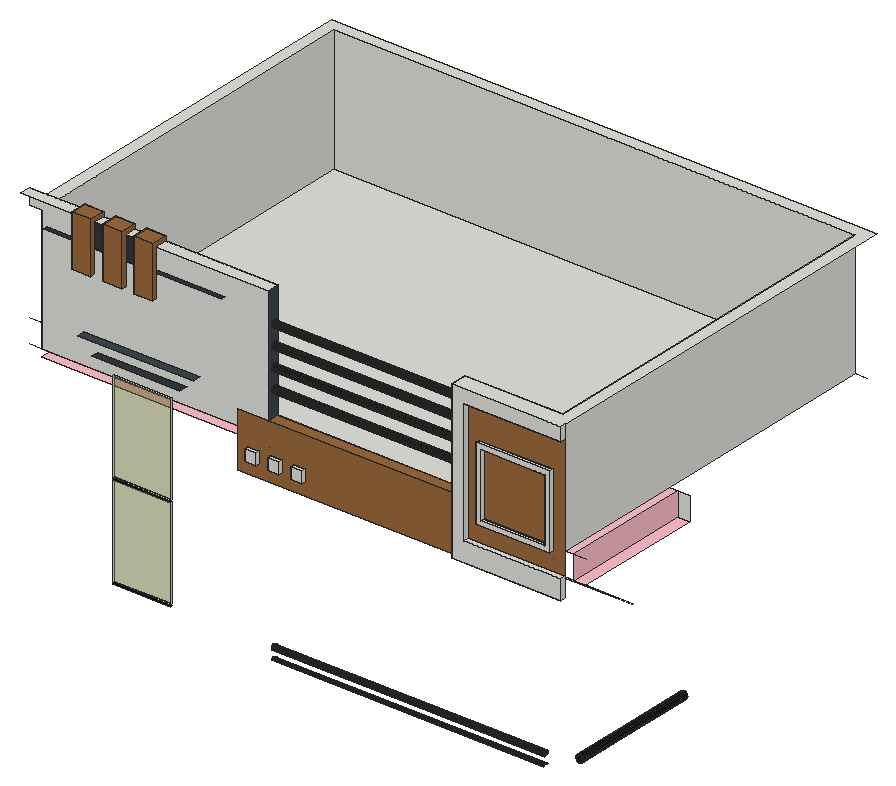
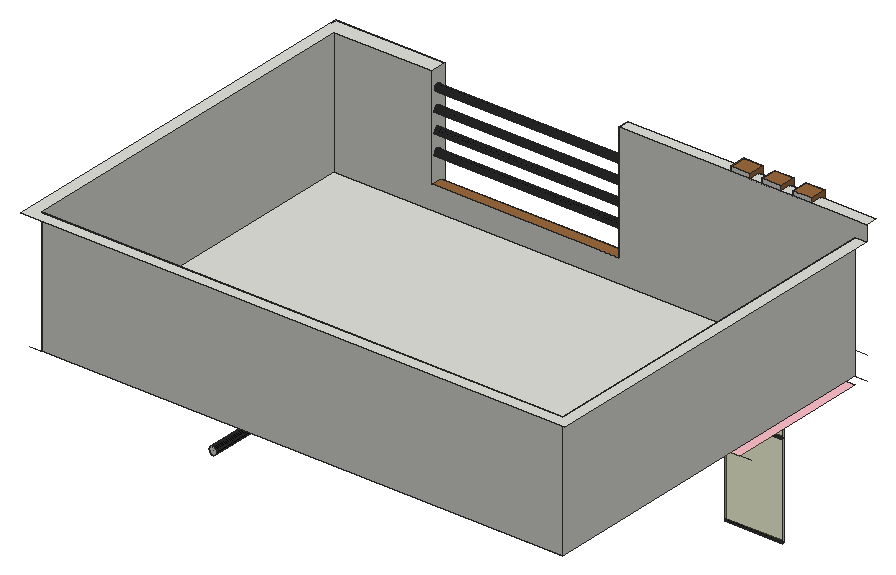
# SketchUp Ruby script. Lengths in inches.
U = 1.inch
M = Sketchup.active_model
def pt(a) = Geom::Point3d.new(a.map { |v| v * U })
def face(e, loops, mat)
  f = e.add_face(loops[0].map { |a| pt(a) })
  loops[1..].each { |l| e.add_face(l.map { |a| pt(a) }).erase! }
  f.material = f.back_material = mat if mat
  f
end
# faces: each face lists its corners as indices into pts; further lists are holes
def faces(e, pts, list, mat = nil) = list.each { |f| face(e, (f[0].is_a?(Array) ? f : [f]).map { |l| l.map { |i| pts[i] } }, mat) }
# xy, xz, yz: faces in a plane at the given z, y or x. An outline is a flat list of corners, or four numbers for a rectangle; further outlines are holes
def ring(l) = l.size == 4 ? [[l[0], l[1]], [l[2], l[1]], [l[2], l[3]], [l[0], l[3]]] : l.each_slice(2).to_a
def flat(e, list, mat, &to3) = list.each { |f| face(e, (f[0].is_a?(Array) ? f : [f]).map { |l| ring(l).map { |u, v| to3.(u, v) } }, mat) }
def xy(e, z, list, mat = nil) = flat(e, list, mat) { |x, y| [x, y, z] }
def xz(e, y, list, mat = nil) = flat(e, list, mat) { |x, z| [x, y, z] }
def yz(e, x, list, mat = nil) = flat(e, list, mat) { |y, z| [x, y, z] }
def lines(e, pts, list) = list.each { |a, b| e.add_line(pt(pts[a]), pt(pts[b])) }
# prism: a flat outline (further loops are holes) pulled along v
def prism(e, loops, v, mat = nil)
  f = face(e, loops, mat); d = Geom::Vector3d.new(v.map { |x| x * U })
  f.pushpull(f.normal.samedirection?(d) ? d.length : -d.length)
end
def box(e, o, s, mat = nil) = prism(e, [[o, [o[0] + s[0], o[1], o[2]], [o[0] + s[0], o[1] + s[1], o[2]], [o[0], o[1] + s[1], o[2]]]], [0, 0, s[2]], mat)
def at(x, y, z, deg = 0) = Geom::Transformation.translation(pt([x, y, z])) * Geom::Transformation.rotation(ORIGIN, Z_AXIS, deg.degrees)
def axes(o, x, y, z) = Geom::Transformation.new([*x, 0, *y, 0, *z, 0, *pt(o).to_a, 1])
def part(name) = M.definitions.add(name)
# library, detail: a bought-in or finely detailed component or shape, given as its bounding box
def library(name, o, s) = part(name).tap { |d| box(d.entities, o, s) }
def detail(e, o, s) = box(e.add_group.entities, o, s)
def put(e, d, t, mat = nil) = e.add_instance(d, t).tap { |i| i.material = mat if mat }
def group(e, t, mat = nil) = e.add_group.tap { |g| g.transformation = t; g.material = mat if mat }.entities
root = M.entities
M.materials.add("[0006_Pink]").color = [255, 192, 203]
M.materials.add("[0111_SlateGray]").color = [49, 56, 63]
M.materials.add("[0111_SlateGray]1").color = [61, 70, 79]
M.materials.add("[0137_Black]").color = [0, 0, 0]
M.materials.add("[Translucent Glass Gray]").color = [124, 128, 62]
M.materials["[Translucent Glass Gray]"].alpha = 0.5
M.materials.add("[Wood Floor]").color = [155, 105, 61]
xy(root,597.83,[[138.3,14,227.59,16]])
xy(root,600.83,[[138.3,14,227.59,16]])
xy(root,682.9,[[411.23,248,466.96,249],[473.67,248,530.59,249],[643.26,248,751.37,249]])
xy(root,741.83,[[138.3,14,227.59,16]])
xy(root,744.83,[[138.3,14,227.59,16]])
xy(root,828,[[821.4375,48.0625,840,248]],"[0006_Pink]")
xy(root,828,[[671.22,0,671.22,8,383.22,8,383.22,26,802.875,26,802.875,8,840,8,840,0]],"[Wood Floor]")
xy(root,847.68,[[350.63,2,368.01,8],[386.32,2,403.69,8],[421.88,2,439.26,8]])
xy(root,858,[[690.42,0,840,8]])
xy(root,864,[[407.75,124.89,404.625,125,401.625,125.91,398.97,127.5625,396.83,129.85,395.35,132.62,394.64,135.67,394.75,138.8,395.66,141.8,397.3125,144.45,399.6,146.59,402.37,148.07,405.42,148.78,408.55,148.67,411.55,147.76,414.2,146.11,416.34,143.82,417.82,141.06,418.53,138,418.42,134.875,417.51,131.875,415.86,129.22,413.57,127.08,410.81,125.6],[527.75,124.89,524.625,125,521.625,125.91,518.97,127.5625,516.83,129.85,515.35,132.62,514.64,135.67,514.75,138.8,515.66,141.8,517.3125,144.45,519.6,146.59,522.37,148.07,525.42,148.78,528.55,148.67,531.55,147.76,534.2,146.11,536.34,143.82,537.82,141.06,538.53,138,538.42,134.875,537.51,131.875,535.86,129.22,533.57,127.08,530.81,125.6],[647.75,124.89,644.625,125,641.625,125.91,638.97,127.5625,636.83,129.85,635.35,132.62,634.64,135.67,634.75,138.8,635.66,141.8,637.3125,144.45,639.6,146.59,642.37,148.07,645.42,148.78,648.55,148.67,651.55,147.76,654.2,146.11,656.34,143.82,657.82,141.06,658.53,138,658.42,134.875,657.51,131.875,655.86,129.22,653.57,127.08,650.81,125.6]])
xy(root,864,[[[18,26,18,248,821.4375,248,821.4375,48.0625,802.875,48.0625,802.875,26],[527.75,124.89,530.81,125.6,533.57,127.08,535.86,129.22,537.51,131.875,538.42,134.875,538.53,138,537.82,141.06,536.34,143.82,534.2,146.11,531.55,147.76,528.55,148.67,525.42,148.78,522.37,148.07,519.6,146.59,517.3125,144.45,515.66,141.8,514.75,138.8,514.64,135.67,515.35,132.62,516.83,129.85,518.97,127.5625,521.625,125.91,524.625,125],[647.75,124.89,650.81,125.6,653.57,127.08,655.86,129.22,657.51,131.875,658.42,134.875,658.53,138,657.82,141.06,656.34,143.82,654.2,146.11,651.55,147.76,648.55,148.67,645.42,148.78,642.37,148.07,639.6,146.59,637.3125,144.45,635.66,141.8,634.75,138.8,634.64,135.67,635.35,132.62,636.83,129.85,638.97,127.5625,641.625,125.91,644.625,125],[407.75,124.89,410.81,125.6,413.57,127.08,415.86,129.22,417.51,131.875,418.42,134.875,418.53,138,417.82,141.06,416.34,143.82,414.2,146.11,411.55,147.76,408.55,148.67,405.42,148.78,402.37,148.07,399.6,146.59,397.3125,144.45,395.66,141.8,394.75,138.8,394.64,135.67,395.35,132.62,396.83,129.85,398.97,127.5625,401.625,125.91,404.625,125]]],"[0006_Pink]")
xy(root,865.06,[[350.63,2,368.01,8],[386.32,2,403.69,8],[421.88,2,439.26,8]])
xy(root,876,[[18,26,822,590]])
xy(root,885.73,[[707.57,2,820.78,8]])
xy(root,885.83,[[138.3,14,227.59,16]])
xy(root,892.8,[[714.64,2,813.7,8]])
xy(root,909.62,[[114.5,2,251.38,14]],"[0111_SlateGray]")
xy(root,912,[[383.22,8,671.22,26]],"[Wood Floor]")
xy(root,930.88,[[93.24,2,272.64,14]],"[0111_SlateGray]1")
xy(root,991.86,[[714.64,2,813.7,8]])
xy(root,998.9375,[[707.57,2,820.78,8]])
xy(root,1020,[[85.01,1,114.04,8],[132.95,1,161.97,8],[180.58,1,209.6,8]])
xy(root,1047.6,[[690.42,0,840,8]])
xy(root,1056,[[36,8,311.22,14]],"[0111_SlateGray]")
xy(root,1068,[[671.22,0,840,0,840,608,0,608,0,26,18,26,18,590,822,590,822,26,671.22,26]])
xy(root,1092,[[0,8,85.01,26],[85.01,8,114.04,26],[114.04,8,132.95,26],[132.95,8,161.97,26],[161.97,8,180.58,26],
  [180.58,8,209.6,26],[209.6,8,383.22,26]])
xy(root,1099,[[85.01,1,114.04,26],[132.95,1,161.97,26],[180.58,1,209.6,26]],"[Wood Floor]")
xz(root,0,[[671.22,828,840,828,840,858,690.42,858,690.42,1047.6,840,1047.6,840,1068,671.22,1068]])
xz(root,1,[[85.01,1020,114.04,1099],[132.95,1020,161.97,1099],[180.58,1020,209.6,1099]],"[Wood Floor]")
xz(root,2,[[350.63,847.68,368.01,865.06],[386.32,847.68,403.69,865.06],[421.88,847.68,439.26,865.06],[[707.57,885.73,820.78,998.9375],[714.64,892.8,813.7,991.86]]])
xz(root,8,[[386.32,847.68,403.69,865.06],[421.88,847.68,439.26,865.06],[[707.57,885.73,820.78,998.9375],[714.64,892.8,813.7,991.86]],[85.01,1020,114.04,1056],[132.95,1020,161.97,1056],
  [180.58,1020,209.6,1056],[85.01,1056,114.04,1092],[132.95,1056,161.97,1092],[180.58,1056,209.6,1092]])
xz(root,8,[[114.04,1056,132.95,1092],[161.97,1056,180.58,1092]],"[0111_SlateGray]")
xz(root,8,[[[335.22,828,671.22,912],[350.63,847.68,368.01,865.06],[386.32,847.68,403.69,865.06],[421.88,847.68,439.26,865.06]],[[690.42,858,840,1047.6],[707.57,885.73,820.78,998.9375]],[714.64,892.8,813.7,991.86]],"[Wood Floor]")
xz(root,14,[[138.3,597.83,227.59,600.83],[138.3,741.83,227.59,744.83]],"[0137_Black]")
xz(root,16,[[138.3,600.83,227.59,741.83],[138.3,744.83,227.59,885.83]],"[Translucent Glass Gray]")
xz(root,26,[[383.22,828,802.875,864],[18,876,18,1068,0,1068,0,1092,383.22,1092,383.22,912,671.22,912,671.22,1068,822,1068,822,876],[85.01,1092,114.04,1099],[132.95,1092,161.97,1099],[180.58,1092,209.6,1099]])
xz(root,248,[[830.72,579.14,829.17,579.35,827.72,579.95,826.48,580.9,825.52,582.14,824.92,583.59,824.72,585.14,824.92,586.7,825.52,588.14,826.48,589.39,827.72,590.34,829.17,590.9375,830.72,591.14,832.27,590.9375,833.72,590.34,834.96,589.39,835.91,588.14,836.51,586.7,836.72,585.14,836.51,583.59,835.91,582.14,834.96,580.9,833.72,579.95,832.27,579.35],[821.4375,828,840,864]])
xz(root,590,[[18,876,822,1068]])
yz(root,18,[[26,876,590,1068]])
yz(root,85.01,[[1,1020,1,1099,26,1099,26,1092,8,1092,8,1020]],"[Wood Floor]")
yz(root,114.04,[[1,1020,8,1020,8,1092,26,1092,26,1099,1,1099]],"[Wood Floor]")
yz(root,132.95,[[1,1020,1,1099,26,1099,26,1092,8,1092,8,1020]],"[Wood Floor]")
yz(root,138.3,[[14,600.83,16,741.83],[14,744.83,16,885.83]])
yz(root,161.97,[[1,1020,8,1020,8,1092,26,1092,26,1099,1,1099]],"[Wood Floor]")
yz(root,180.58,[[1,1020,1,1099,26,1099,26,1092,8,1092,8,1020]],"[Wood Floor]")
yz(root,209.6,[[1,1020,8,1020,8,1092,26,1092,26,1099,1,1099]],"[Wood Floor]")
yz(root,227.59,[[14,600.83,16,741.83],[14,744.83,16,885.83]])
yz(root,350.63,[[2,847.68,8,865.06]])
yz(root,368.01,[[2,847.68,8,865.06]])
yz(root,383.22,[[17.13,592.37,16.09,592.47,15.11,592.84,14.26,593.45,13.6,594.26,13.17,595.21,13,596.24,13.1,597.28,13.47,598.25,14.08,599.1,14.89,599.76,15.84,600.2,16.87,600.36,17.91,600.26,18.89,599.89,19.74,599.28,20.4,598.48,20.83,597.53,21,596.49,20.9,595.46,20.53,594.48,19.92,593.63,19.11,592.97,18.16,592.54]])
yz(root,383.22,[[[8,912,26,1092],[17.14,1037.85,15.84,1037.98,14.625,1038.45,13.57,1039.21,12.74,1040.22,12.21,1041.42,12,1042.7,12.14,1044,12.6,1045.22,13.37,1046.28,14.38,1047.1,15.57,1047.64,16.86,1047.84,18.16,1047.71,19.375,1047.24,20.43,1046.48,21.26,1045.47,21.79,1044.28,22,1042.99,21.86,1041.6875,21.4,1040.47,20.63,1039.41,19.62,1038.59,18.43,1038.05],[17.14,1007.85,15.84,1007.98,14.625,1008.45,13.57,1009.21,12.74,1010.22,12.21,1011.42,12,1012.7,12.14,1014,12.6,1015.22,13.37,1016.28,14.38,1017.1,15.57,1017.64,16.86,1017.84,18.16,1017.71,19.375,1017.24,20.43,1016.48,21.26,1015.47,21.79,1014.28,22,1012.99,21.86,1011.6875,21.4,1010.47,20.63,1009.41,19.62,1008.59,18.43,1008.05],[17.14,977.85,15.84,977.98,14.625,978.45,13.57,979.21,12.74,980.22,12.21,981.42,12,982.7,12.14,984,12.6,985.22,13.37,986.28,14.38,987.1,15.57,987.64,16.86,987.84,18.16,987.71,19.375,987.24,20.43,986.48,21.26,985.47,21.79,984.28,22,982.99,21.86,981.6875,21.4,980.47,20.63,979.41,19.62,978.59,18.43,978.05],[17.14,947.85,15.84,947.98,14.625,948.45,13.57,949.21,12.74,950.22,12.21,951.42,12,952.7,12.14,954,12.6,955.22,13.37,956.28,14.38,957.1,15.57,957.64,16.86,957.84,18.16,957.71,19.375,957.24,20.43,956.48,21.26,955.47,21.79,954.28,22,952.99,21.86,951.6875,21.4,950.47,20.63,949.41,19.62,948.59,18.43,948.05]]],"[0111_SlateGray]1")
yz(root,386.32,[[2,847.68,8,865.06]])
yz(root,403.69,[[2,847.68,8,865.06]])
yz(root,421.88,[[2,847.68,8,865.06]])
yz(root,439.26,[[2,847.68,8,865.06]])
yz(root,671.22,[[[0,828,0,1068,26,1068,26,912,8,912,8,828],[17.14,1037.85,18.43,1038.05,19.62,1038.59,20.63,1039.41,21.4,1040.47,21.86,1041.6875,22,1042.99,21.79,1044.28,21.26,1045.47,20.43,1046.48,19.375,1047.24,18.16,1047.71,16.86,1047.84,15.57,1047.64,14.38,1047.1,13.37,1046.28,12.6,1045.22,12.14,1044,12,1042.7,12.21,1041.42,12.74,1040.22,13.57,1039.21,14.625,1038.45,15.84,1037.98],[17.14,977.85,18.43,978.05,19.62,978.59,20.63,979.41,21.4,980.47,21.86,981.6875,22,982.99,21.79,984.28,21.26,985.47,20.43,986.48,19.375,987.24,18.16,987.71,16.86,987.84,15.57,987.64,14.38,987.1,13.37,986.28,12.6,985.22,12.14,984,12,982.7,12.21,981.42,12.74,980.22,13.57,979.21,14.625,978.45,15.84,977.98],[17.14,1007.85,18.43,1008.05,19.62,1008.59,20.63,1009.41,21.4,1010.47,21.86,1011.6875,22,1012.99,21.79,1014.28,21.26,1015.47,20.43,1016.48,19.375,1017.24,18.16,1017.71,16.86,1017.84,15.57,1017.64,14.38,1017.1,13.37,1016.28,12.6,1015.22,12.14,1014,12,1012.7,12.21,1011.42,12.74,1010.22,13.57,1009.21,14.625,1008.45,15.84,1007.98],[17.14,947.85,18.43,948.05,19.62,948.59,20.63,949.41,21.4,950.47,21.86,951.6875,22,952.99,21.79,954.28,21.26,955.47,20.43,956.48,19.375,957.24,18.16,957.71,16.86,957.84,15.57,957.64,14.38,957.1,13.37,956.28,12.6,955.22,12.14,954,12,952.7,12.21,951.42,12.74,950.22,13.57,949.21,14.625,948.45,15.84,947.98]],[17.14,947.85,18.43,948.05,19.62,948.59,20.63,949.41,21.4,950.47,21.86,951.6875,22,952.99,21.79,954.28,21.26,955.47,20.43,956.48,19.375,957.24,18.16,957.71,16.86,957.84,15.57,957.64,14.38,957.1,13.37,956.28,12.6,955.22,12.14,954,12,952.7,12.21,951.42,12.74,950.22,13.57,949.21,14.625,948.45,15.84,947.98],[17.14,977.85,18.43,978.05,19.62,978.59,20.63,979.41,21.4,980.47,21.86,981.6875,22,982.99,21.79,984.28,21.26,985.47,20.43,986.48,19.375,987.24,18.16,987.71,16.86,987.84,15.57,987.64,14.38,987.1,13.37,986.28,12.6,985.22,12.14,984,12,982.7,12.21,981.42,12.74,980.22,13.57,979.21,14.625,978.45,15.84,977.98],[17.14,1007.85,18.43,1008.05,19.62,1008.59,20.63,1009.41,21.4,1010.47,21.86,1011.6875,22,1012.99,21.79,1014.28,21.26,1015.47,20.43,1016.48,19.375,1017.24,18.16,1017.71,16.86,1017.84,15.57,1017.64,14.38,1017.1,13.37,1016.28,12.6,1015.22,12.14,1014,12,1012.7,12.21,1011.42,12.74,1010.22,13.57,1009.21,14.625,1008.45,15.84,1007.98],[17.14,1037.85,18.43,1038.05,19.62,1038.59,20.63,1039.41,21.4,1040.47,21.86,1041.6875,22,1042.99,21.79,1044.28,21.26,1045.47,20.43,1046.48,19.375,1047.24,18.16,1047.71,16.86,1047.84,15.57,1047.64,14.38,1047.1,13.37,1046.28,12.6,1045.22,12.14,1044,12,1042.7,12.21,1041.42,12.74,1040.22,13.57,1039.21,14.625,1038.45,15.84,1037.98]])
yz(root,690.42,[[0,858,8,1047.6]])
yz(root,707.57,[[2,885.73,8,998.9375]])
yz(root,714.64,[[2,892.8,8,991.86]])
yz(root,813.7,[[2,892.8,8,991.86]])
yz(root,820.78,[[2,885.73,8,998.9375]])
yz(root,821.4375,[[48.0625,828,248,864]],"[0006_Pink]")
yz(root,822,[[26,876,590,1068]])
yz(root,840,[[0,828,8,858],[0,1047.6,8,1068]])
p = [[829.17,248,579.35],[830.72,248,579.14],[830.72,48.0625,579.14],[829.17,48.0625,579.35],[832.27,248,579.35],[832.27,48.0625,579.35],
  [383.22,13.47,580.25],[383.22,13.1,579.28],[802.875,13.1,579.28],[802.875,13.47,580.25],[827.72,248,579.95],[827.72,48.0625,579.95],
  [833.72,248,579.95],[833.72,48.0625,579.95],[383.22,20.83,579.53],[383.22,20.4,580.48],[802.875,20.4,580.48],[802.875,20.83,579.53],
  [826.48,248,580.9],[826.48,48.0625,580.9],[834.96,248,580.9],[834.96,48.0625,580.9],[383.22,14.08,581.1],[802.875,14.08,581.1],
  [383.22,19.74,581.28],[802.875,19.74,581.28],[825.52,248,582.14],[825.52,48.0625,582.14],[835.91,248,582.14],[835.91,48.0625,582.14],
  [383.22,14.89,581.76],[802.875,14.89,581.76],[383.22,18.89,581.89],[802.875,18.89,581.89],[383.22,15.84,582.2],[802.875,15.84,582.2],
  [383.22,17.91,582.26],[802.875,17.91,582.26],[824.92,248,583.59],[824.92,48.0625,583.59],[836.51,248,583.59],[836.51,48.0625,583.59],
  [383.22,16.87,582.36],[802.875,16.87,582.36],[824.72,248,585.14],[824.72,48.0625,585.14],[836.72,248,585.14],[836.72,48.0625,585.14],
  [824.92,248,586.7],[824.92,48.0625,586.7],[836.51,248,586.7],[836.51,48.0625,586.7],[825.52,248,588.14],[825.52,48.0625,588.14],
  [835.91,248,588.14],[835.91,48.0625,588.14],[826.48,248,589.39],[826.48,48.0625,589.39],[834.96,248,589.39],[834.96,48.0625,589.39],
  [827.72,248,590.34],[827.72,48.0625,590.34],[833.72,248,590.34],[833.72,48.0625,590.34],[829.17,248,590.9375],[829.17,48.0625,590.9375],
  [832.27,248,590.9375],[832.27,48.0625,590.9375],[830.72,248,591.14],[830.72,48.0625,591.14],[383.22,16.09,592.47],[383.22,17.13,592.37],
  [802.875,17.13,592.37],[802.875,16.09,592.47],[383.22,18.16,592.54],[802.875,18.16,592.54],[383.22,15.11,592.84],[802.875,15.11,592.84],
  [383.22,19.11,592.97],[802.875,19.11,592.97],[383.22,14.26,593.45],[802.875,14.26,593.45],[383.22,19.92,593.63],[802.875,19.92,593.63],
  [383.22,13.6,594.26],[802.875,13.6,594.26],[383.22,20.53,594.48],[802.875,20.53,594.48],[383.22,13.17,595.21],[802.875,13.17,595.21],
  [383.22,20.9,595.46],[802.875,20.9,595.46],[383.22,13,596.24],[802.875,13,596.24],[383.22,21,596.49],[802.875,21,596.49],
  [383.22,13.1,597.28],[802.875,13.1,597.28],[383.22,20.83,597.53],[802.875,20.83,597.53],[383.22,13.47,598.25],[802.875,13.47,598.25],
  [383.22,20.4,598.48],[802.875,20.4,598.48],[383.22,14.08,599.1],[802.875,14.08,599.1],[383.22,19.74,599.28],[802.875,19.74,599.28],
  [383.22,14.89,599.76],[802.875,14.89,599.76],[383.22,18.89,599.89],[802.875,18.89,599.89],[383.22,15.84,600.2],[802.875,15.84,600.2],
  [383.22,17.91,600.26],[802.875,17.91,600.26],[383.22,16.87,600.36],[802.875,16.87,600.36],[671.22,17.14,947.85],[671.22,15.84,947.98],
  [383.22,15.84,947.98],[383.22,17.14,947.85],[671.22,18.43,948.05],[383.22,18.43,948.05],[671.22,14.625,948.45],[383.22,14.625,948.45],
  [671.22,19.62,948.59],[383.22,19.62,948.59],[671.22,13.57,949.21],[383.22,13.57,949.21],[671.22,20.63,949.41],[383.22,20.63,949.41],
  [671.22,12.74,950.22],[383.22,12.74,950.22],[671.22,21.4,950.47],[383.22,21.4,950.47],[671.22,12.21,951.42],[383.22,12.21,951.42],
  [671.22,21.86,951.6875],[383.22,21.86,951.6875],[671.22,12,952.7],[383.22,12,952.7],[671.22,22,952.99],[383.22,22,952.99],
  [671.22,12.14,954],[383.22,12.14,954],[671.22,21.79,954.28],[383.22,21.79,954.28],[671.22,12.6,955.22],[383.22,12.6,955.22],
  [671.22,21.26,955.47],[383.22,21.26,955.47],[671.22,13.37,956.28],[383.22,13.37,956.28],[671.22,20.43,956.48],[383.22,20.43,956.48],
  [671.22,14.38,957.1],[383.22,14.38,957.1],[671.22,19.375,957.24],[383.22,19.375,957.24],[671.22,15.57,957.64],[383.22,15.57,957.64],
  [671.22,18.16,957.71],[383.22,18.16,957.71],[671.22,16.86,957.84],[383.22,16.86,957.84],[671.22,17.14,977.85],[671.22,15.84,977.98],
  [383.22,15.84,977.98],[383.22,17.14,977.85],[671.22,18.43,978.05],[383.22,18.43,978.05],[671.22,14.625,978.45],[383.22,14.625,978.45],
  [671.22,19.62,978.59],[383.22,19.62,978.59],[671.22,13.57,979.21],[383.22,13.57,979.21],[671.22,20.63,979.41],[383.22,20.63,979.41],
  [671.22,12.74,980.22],[383.22,12.74,980.22],[671.22,21.4,980.47],[383.22,21.4,980.47],[671.22,12.21,981.42],[383.22,12.21,981.42],
  [671.22,21.86,981.6875],[383.22,21.86,981.6875],[671.22,12,982.7],[383.22,12,982.7],[671.22,22,982.99],[383.22,22,982.99],
  [671.22,12.14,984],[383.22,12.14,984],[671.22,21.79,984.28],[383.22,21.79,984.28],[671.22,12.6,985.22],[383.22,12.6,985.22],
  [671.22,21.26,985.47],[383.22,21.26,985.47],[671.22,13.37,986.28],[383.22,13.37,986.28],[671.22,20.43,986.48],[383.22,20.43,986.48],
  [671.22,14.38,987.1],[383.22,14.38,987.1],[671.22,19.375,987.24],[383.22,19.375,987.24],[671.22,15.57,987.64],[383.22,15.57,987.64],
  [671.22,18.16,987.71],[383.22,18.16,987.71],[671.22,16.86,987.84],[383.22,16.86,987.84],[671.22,17.14,1007.85],[671.22,15.84,1007.98],
  [383.22,15.84,1007.98],[383.22,17.14,1007.85],[671.22,18.43,1008.05],[383.22,18.43,1008.05],[671.22,14.625,1008.45],[383.22,14.625,1008.45],
  [671.22,19.62,1008.59],[383.22,19.62,1008.59],[671.22,13.57,1009.21],[383.22,13.57,1009.21],[671.22,20.63,1009.41],[383.22,20.63,1009.41],
  [671.22,12.74,1010.22],[383.22,12.74,1010.22],[671.22,21.4,1010.47],[383.22,21.4,1010.47],[671.22,12.21,1011.42],[383.22,12.21,1011.42],
  [671.22,21.86,1011.6875],[383.22,21.86,1011.6875],[671.22,12,1012.7],[383.22,12,1012.7],[671.22,22,1012.99],[383.22,22,1012.99],
  [671.22,12.14,1014],[383.22,12.14,1014],[671.22,21.79,1014.28],[383.22,21.79,1014.28],[671.22,12.6,1015.22],[383.22,12.6,1015.22],
  [671.22,21.26,1015.47],[383.22,21.26,1015.47],[671.22,13.37,1016.28],[383.22,13.37,1016.28],[671.22,20.43,1016.48],[383.22,20.43,1016.48],
  [671.22,14.38,1017.1],[383.22,14.38,1017.1],[671.22,19.375,1017.24],[383.22,19.375,1017.24],[671.22,15.57,1017.64],[383.22,15.57,1017.64],
  [671.22,18.16,1017.71],[383.22,18.16,1017.71],[671.22,16.86,1017.84],[383.22,16.86,1017.84],[671.22,17.14,1037.85],[671.22,15.84,1037.98],
  [383.22,15.84,1037.98],[383.22,17.14,1037.85],[671.22,18.43,1038.05],[383.22,18.43,1038.05],[671.22,14.625,1038.45],[383.22,14.625,1038.45],
  [671.22,19.62,1038.59],[383.22,19.62,1038.59],[671.22,13.57,1039.21],[383.22,13.57,1039.21],[671.22,20.63,1039.41],[383.22,20.63,1039.41],
  [671.22,12.74,1040.22],[383.22,12.74,1040.22],[671.22,21.4,1040.47],[383.22,21.4,1040.47],[671.22,12.21,1041.42],[383.22,12.21,1041.42],
  [671.22,21.86,1041.6875],[383.22,21.86,1041.6875],[671.22,12,1042.7],[383.22,12,1042.7],[671.22,22,1042.99],[383.22,22,1042.99],
  [671.22,12.14,1044],[383.22,12.14,1044],[671.22,21.79,1044.28],[383.22,21.79,1044.28],[671.22,12.6,1045.22],[383.22,12.6,1045.22],
  [671.22,21.26,1045.47],[383.22,21.26,1045.47],[671.22,13.37,1046.28],[383.22,13.37,1046.28],[671.22,20.43,1046.48],[383.22,20.43,1046.48],
  [671.22,14.38,1047.1],[383.22,14.38,1047.1],[671.22,19.375,1047.24],[383.22,19.375,1047.24],[671.22,15.57,1047.64],[383.22,15.57,1047.64],
  [671.22,18.16,1047.71],[383.22,18.16,1047.71],[671.22,16.86,1047.84],[383.22,16.86,1047.84],[822,590,876],[840,590,876],
  [822,8,876],[822,26,876],[18,248,864],[0,248,864],[840,48.0625,864],[821.4375,48.0625,864],
  [383.22,26,864],[383.22,8,864],[802.875,26,864],[802.875,8,864],[383.22,8,876],[383.22,26,876],
  [18,26,876],[0,26,876],[18,26,912],[0,26,912],[671.22,17,952.85],[383.22,17,952.85],
  [671.22,17,982.85],[383.22,17,982.85],[671.22,17,1012.85],[383.22,17,1012.85],[671.22,17,1042.85],[383.22,17,1042.85],
  [383.22,17,596.37],[802.875,17,596.37],[830.72,248,585.14],[830.72,48.0625,585.14]]
faces(root,p,[[0,1,2,3],[1,4,5,2],[6,7,8,9],[10,0,3,11],[4,12,13,5],[14,15,16,17],[18,10,11,19],[12,20,21,13],
  [22,6,9,23],[15,24,25,16],[26,18,19,27],[20,28,29,21],[30,22,23,31],[24,32,33,25],[34,30,31,35],[32,36,37,33],
  [38,26,27,39],[28,40,41,29],[42,34,35,43],[36,42,43,37],[44,38,39,45],[40,46,47,41],[48,44,45,49],[46,50,51,47],
  [52,48,49,53],[50,54,55,51],[56,52,53,57],[54,58,59,55],[60,56,57,61],[58,62,63,59],[64,60,61,65],[62,66,67,63],
  [68,64,65,69],[66,68,69,67],[70,71,72,73],[71,74,75,72],[76,70,73,77],[74,78,79,75],[80,76,77,81],[78,82,83,79],
  [84,80,81,85],[82,86,87,83],[88,84,85,89],[86,90,91,87],[92,88,89,93],[90,94,95,91],[96,92,93,97],[94,98,99,95],
  [100,96,97,101],[98,102,103,99],[104,100,101,105],[102,106,107,103],[108,104,105,109],[106,110,111,107],[112,108,109,113],[110,114,115,111],
  [116,112,113,117],[114,116,117,115],[118,119,120,121],[122,118,121,123],[119,124,125,120],[126,122,123,127],[124,128,129,125],[130,126,127,131],
  [128,132,133,129],[134,130,131,135],[132,136,137,133],[138,134,135,139],[136,140,141,137],[142,138,139,143],[140,144,145,141],[146,142,143,147],
  [144,148,149,145],[150,146,147,151],[148,152,153,149],[154,150,151,155],[152,156,157,153],[158,154,155,159],[156,160,161,157],[162,158,159,163],
  [160,164,165,161],[164,162,163,165],[166,167,168,169],[170,166,169,171],[167,172,173,168],[174,170,171,175],[172,176,177,173],[178,174,175,179],
  [176,180,181,177],[182,178,179,183],[180,184,185,181],[186,182,183,187],[184,188,189,185],[190,186,187,191],[188,192,193,189],[194,190,191,195],
  [192,196,197,193],[198,194,195,199],[196,200,201,197],[202,198,199,203],[200,204,205,201],[206,202,203,207],[204,208,209,205],[210,206,207,211],
  [208,212,213,209],[212,210,211,213],[214,215,216,217],[218,214,217,219],[215,220,221,216],[222,218,219,223],[220,224,225,221],[226,222,223,227],
  [224,228,229,225],[230,226,227,231],[228,232,233,229],[234,230,231,235],[232,236,237,233],[238,234,235,239],[236,240,241,237],[242,238,239,243],
  [240,244,245,241],[246,242,243,247],[244,248,249,245],[250,246,247,251],[248,252,253,249],[254,250,251,255],[252,256,257,253],[258,254,255,259],
  [256,260,261,257],[260,258,259,261],[262,263,264,265],[266,262,265,267],[263,268,269,264],[270,266,267,271],[268,272,273,269],[274,270,271,275],
  [272,276,277,273],[278,274,275,279],[276,280,281,277],[282,278,279,283],[280,284,285,281],[286,282,283,287],[284,288,289,285],[290,286,287,291],
  [288,292,293,289],[294,290,291,295],[292,296,297,293],[298,294,295,299],[296,300,301,297],[302,298,299,303],[300,304,305,301],[306,302,303,307],
  [304,308,309,305],[308,306,307,309]],"[0137_Black]")
lines(root,p,[[310,311],[312,313],[314,315],[316,317],[318,319],[320,321],[322,323],[324,325],[326,327],[328,329],[330,331],[332,333],
  [334,335],[336,337],[338,339]])
